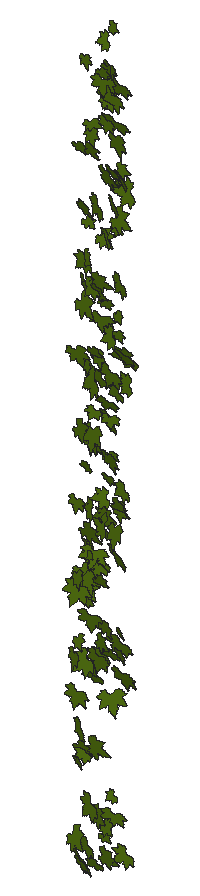
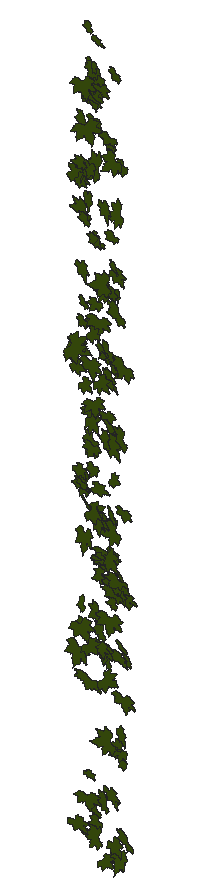
# SketchUp Ruby script. Lengths in inches.
U = 1.inch
M = Sketchup.active_model
def pt(a) = Geom::Point3d.new(a.map { |v| v * U })
def face(e, loops, mat)
  f = e.add_face(loops[0].map { |a| pt(a) })
  loops[1..].each { |l| e.add_face(l.map { |a| pt(a) }).erase! }
  f.material = f.back_material = mat if mat
  f
end
# faces: each face lists its corners as indices into pts; further lists are holes
def faces(e, pts, list, mat = nil) = list.each { |f| face(e, (f[0].is_a?(Array) ? f : [f]).map { |l| l.map { |i| pts[i] } }, mat) }
# xy, xz, yz: faces in a plane at the given z, y or x. An outline is a flat list of corners, or four numbers for a rectangle; further outlines are holes
def ring(l) = l.size == 4 ? [[l[0], l[1]], [l[2], l[1]], [l[2], l[3]], [l[0], l[3]]] : l.each_slice(2).to_a
def flat(e, list, mat, &to3) = list.each { |f| face(e, (f[0].is_a?(Array) ? f : [f]).map { |l| ring(l).map { |u, v| to3.(u, v) } }, mat) }
def xy(e, z, list, mat = nil) = flat(e, list, mat) { |x, y| [x, y, z] }
def xz(e, y, list, mat = nil) = flat(e, list, mat) { |x, z| [x, y, z] }
def yz(e, x, list, mat = nil) = flat(e, list, mat) { |y, z| [x, y, z] }
def lines(e, pts, list) = list.each { |a, b| e.add_line(pt(pts[a]), pt(pts[b])) }
# prism: a flat outline (further loops are holes) pulled along v
def prism(e, loops, v, mat = nil)
  f = face(e, loops, mat); d = Geom::Vector3d.new(v.map { |x| x * U })
  f.pushpull(f.normal.samedirection?(d) ? d.length : -d.length)
end
def box(e, o, s, mat = nil) = prism(e, [[o, [o[0] + s[0], o[1], o[2]], [o[0] + s[0], o[1] + s[1], o[2]], [o[0], o[1] + s[1], o[2]]]], [0, 0, s[2]], mat)
def at(x, y, z, deg = 0) = Geom::Transformation.translation(pt([x, y, z])) * Geom::Transformation.rotation(ORIGIN, Z_AXIS, deg.degrees)
def axes(o, x, y, z) = Geom::Transformation.new([*x, 0, *y, 0, *z, 0, *pt(o).to_a, 1])
def part(name) = M.definitions.add(name)
# library, detail: a bought-in or finely detailed component or shape, given as its bounding box
def library(name, o, s) = part(name).tap { |d| box(d.entities, o, s) }
def detail(e, o, s) = box(e.add_group.entities, o, s)
def put(e, d, t, mat = nil) = e.add_instance(d, t).tap { |i| i.material = mat if mat }
def group(e, t, mat = nil) = e.add_group.tap { |g| g.transformation = t; g.material = mat if mat }.entities
root = M.entities
M.materials.add("[Vegetation Blur 03]").color = [83, 114, 18]
c1 = part("ivy")
xy(c1.entities,0,[[0.782,0,0.786,0,0.787,0.005,0.789,0.009,0.821,0.072,0.875,0.147,1.001,0.272,1.073,0.331,1.137,0.363,1.178,0.379,1.223,0.384,1.272,0.383,1.311,0.374,1.36,0.355,1.399,0.334,1.491,0.285,1.541,0.244,1.583,0.199,1.617,0.15,1.64,0.128,1.662,0.115,1.717,0.105,1.745,0.093,1.784,0.054,1.819,0.057,1.854,0.064,1.882,0.075,1.896,0.074,1.91,0.071,1.937,0.063,1.964,0.053,1.99,0.038,2.016,0.015,2.034,0.002,2.04,0,2.038,0.003,2.036,0.007,2.033,0.038,2.036,0.068,2.045,0.1,2.055,0.116,2.064,0.123,2.077,0.129,2.088,0.129,2.106,0.132,2.118,0.13,2.179,0.132,2.207,0.133,2.225,0.133,2.242,0.138,2.22,0.162,2.207,0.186,2.206,0.213,2.212,0.236,2.228,0.262,2.247,0.274,2.298,0.283,2.355,0.294,2.37,0.296,2.376,0.295,2.377,0.3,2.377,0.303,2.385,0.329,2.411,0.37,2.426,0.392,2.449,0.407,2.511,0.426,2.561,0.444,2.619,0.466,2.589,0.469,2.561,0.476,2.501,0.5,2.449,0.516,2.424,0.523,2.401,0.535,2.377,0.556,2.372,0.568,2.36,0.575,2.268,0.586,2.225,0.592,2.207,0.599,2.194,0.61,2.143,0.65,2.13,0.664,2.122,0.682,2.123,0.7,2.13,0.719,2.148,0.75,2.17,0.781,2.195,0.807,2.221,0.828,2.284,0.874,2.291,0.88,2.288,0.887,2.276,0.9,2.267,0.916,2.265,0.933,2.273,0.967,2.292,1.002,2.313,1.03,2.334,1.054,2.348,1.067,2.358,1.074,2.363,1.076,2.362,1.081,2.35,1.094,2.347,1.11,2.35,1.143,2.359,1.18,2.385,1.254,2.415,1.324,2.448,1.393,2.45,1.4,2.446,1.398,2.44,1.394,2.427,1.383,2.402,1.36,2.376,1.339,2.345,1.324,2.305,1.309,2.282,1.303,2.273,1.306,2.245,1.294,2.212,1.287,2.187,1.291,2.163,1.301,2.142,1.316,2.134,1.327,2.124,1.325,2.09,1.292,2.053,1.259,2.014,1.234,1.973,1.215,1.954,1.21,1.931,1.208,1.909,1.212,1.893,1.22,1.879,1.233,1.872,1.248,1.867,1.281,1.864,1.319,1.821,1.258,1.773,1.197,1.726,1.141,1.698,1.121,1.679,1.116,1.666,1.117,1.647,1.122,1.632,1.129,1.62,1.141,1.617,1.154,1.617,1.219,1.621,1.254,1.623,1.268,1.623,1.281,1.618,1.314,1.606,1.346,1.603,1.375,1.607,1.403,1.603,1.467,1.599,1.499,1.605,1.525,1.614,1.552,1.629,1.577,1.635,1.589,1.629,1.587,1.618,1.582,1.596,1.566,1.581,1.556,1.568,1.552,1.557,1.55,1.545,1.553,1.531,1.562,1.522,1.572,1.504,1.591,1.486,1.611,1.474,1.631,1.457,1.666,1.455,1.684,1.457,1.698,1.452,1.715,1.444,1.728,1.424,1.754,1.419,1.772,1.423,1.786,1.434,1.819,1.444,1.848,1.446,1.855,1.44,1.861,1.43,1.867,1.386,1.904,1.349,1.948,1.326,1.973,1.31,1.995,1.288,2.048,1.284,2.153,1.287,2.254,1.284,2.255,1.282,2.253,1.278,2.247,1.274,2.237,1.266,2.216,1.226,2.125,1.208,2.076,1.184,2.033,1.155,1.984,1.135,1.942,1.111,1.899,1.083,1.861,1.053,1.85,1.059,1.83,1.061,1.809,1.056,1.79,1.049,1.767,1.04,1.749,1.018,1.733,0.994,1.726,0.942,1.734,0.95,1.6875,0.944,1.645,0.932,1.608,0.911,1.585,0.881,1.58,0.854,1.582,0.828,1.588,0.785,1.618,0.773,1.625,0.775,1.614,0.779,1.598,0.796,1.502,0.818,1.402,0.861,1.283,0.882,1.224,0.894,1.174,0.892,1.148,0.886,1.123,0.881,1.107,0.872,1.099,0.849,1.094,0.818,1.092,0.789,1.098,0.762,1.107,0.753,1.113,0.721,1.139,0.698,1.163,0.678,1.194,0.665,1.224,0.628,1.28,0.612,1.312,0.606,1.327,0.606,1.314,0.599,1.282,0.594,1.267,0.581,1.256,0.544,1.245,0.512,1.244,0.473,1.249,0.444,1.256,0.382,1.288,0.339,1.306,0.324,1.316,0.317,1.324,0.309,1.326,0.27,1.314,0.227,1.313,0.185,1.3125,0.152,1.317,0.122,1.328,0.092,1.345,0.073,1.353,0.079,1.338,0.092,1.308,0.117,1.249,0.13,1.215,0.139,1.164,0.147,1.148,0.157,1.136,0.163,1.122,0.174,1.086,0.177,1.067,0.182,1.054,0.186,1.043,0.191,1.038,0.211,1.028,0.237,1.005,0.25,0.974,0.253,0.96,0.25,0.944,0.242,0.914,0.243,0.906,0.249,0.902,0.26,0.894,0.289,0.88,0.307,0.873,0.322,0.862,0.364,0.799,0.403,0.738,0.431,0.709,0.439,0.691,0.441,0.678,0.4375,0.66,0.428,0.645,0.394,0.623,0.303,0.594,0.255,0.581,0.214,0.577,0.179,0.573,0.173,0.568,0.175,0.561,0.167,0.55,0.141,0.523,0.113,0.503,0.077,0.49,0.045,0.486,0.026,0.485,0.019,0.486,0.011,0.483,0,0.471,0.014,0.467,0.044,0.455,0.058,0.447,0.07,0.438,0.097,0.411,0.125,0.394,0.158,0.377,0.174,0.366,0.182,0.359,0.185,0.361,0.242,0.331,0.253,0.316,0.258,0.303,0.262,0.283,0.274,0.278,0.308,0.274,0.341,0.252,0.366,0.226,0.366,0.222,0.37,0.22,0.38,0.221,0.395,0.221,0.425,0.216,0.45,0.207,0.465,0.192,0.473,0.178,0.484,0.15,0.489,0.116,0.483,0.089,0.468,0.058,0.45,0.035,0.435,0.018,0.429,0.011,0.434,0.012,0.438,0.014,0.469,0.019,0.542,0.016,0.581,0.015,0.612,0.027,0.68,0.055,0.696,0.057,0.712,0.052,0.73,0.045,0.741,0.036,0.766,0.014]])
put(root,c1,axes([72.84,173.7,61.72],[0.32192,-0.21102,-0.29136],[-0.33943,0.22769,-0.27574],[-0.15085,-0.96265,-0.00135]),"[Vegetation Blur 03]")
put(root,c1,axes([72.2,173.7,63.29],[0.58789,-0.11281,-0.04556],[-0.05859,-0.05769,-0.48112],[-0.05185,-1.21383,0.0271]),"[Vegetation Blur 03]")
put(root,c1,axes([72.33,173.7,72.92],[0.43658,-0.10423,0.00392],[0.00224,-0.04583,-0.35826],[-0.05083,-0.89729,0.01784]),"[Vegetation Blur 03]")
put(root,c1,axes([72.26,173.7,68.72],[0.62885,-0.10059,-0.07918],[-0.103,-0.17922,-0.50906],[-0.03454,-1.29703,0.07648]),"[Vegetation Blur 03]")
put(root,c1,axes([72.38,173.7,65.2],[0.43914,-0.29657,0.03896],[0.03337,-0.10478,-0.37595],[-0.14811,-0.90294,0.03083]),"[Vegetation Blur 03]")
put(root,c1,axes([72.09,173.7,55.21],[0.24806,0.03915,0.43187],[0.51673,-0.28046,-0.19369],[-0.11561,-1.16947,0.06091]),"[Vegetation Blur 03]")
put(root,c1,axes([72.89,173.7,68.78],[0.30881,-0.07275,-0.21101],[-0.25864,0.02403,-0.25343],[-0.03462,-0.82843,0.01118]),"[Vegetation Blur 03]")
put(root,c1,axes([72.42,173.7,90.69],[0.29342,-0.08692,0.17033],[0.21238,0.06683,-0.23833],[-0.01533,-0.73794,-0.04165]),"[Vegetation Blur 03]")
put(root,c1,axes([72.03,173.7,80.21],[0.52256,-0.08904,0.24501],[0.30058,-0.01277,-0.42774],[-0.04062,-1.24009,-0.01319]),"[Vegetation Blur 03]")
put(root,c1,axes([72.53,173.7,59.625],[0.27556,-0.19726,0.13683],[0.17351,-0.01114,-0.23526],[-0.08482,-0.66366,-0.03672]),"[Vegetation Blur 03]")
put(root,c1,axes([72.5,173.7,65.52],[0.23663,-0.00308,0.21961],[0.25991,-0.18831,-0.18695],[-0.06967,-0.71292,0.04843]),"[Vegetation Blur 03]")
put(root,c1,axes([73.38,173.7,74.76],[0.04516,0.08728,-0.24004],[-0.29622,0.06188,-0.03358],[-0.02362,-0.6092,-0.0378]),"[Vegetation Blur 03]")
put(root,c1,axes([72.97,173.7,85.52],[0.38178,-0.11889,-0.25625],[-0.31299,0.05919,-0.31491],[-0.06294,-1.01546,0.01165]),"[Vegetation Blur 03]")
put(root,c1,axes([73.13,173.7,55.86],[0.3336,-0.07994,-0.30777],[-0.37102,0.14358,-0.27372],[-0.07791,-1.02608,-0.01433]),"[Vegetation Blur 03]")
put(root,c1,axes([73.05,173.7,84.32],[0.23472,-0.16453,-0.13977],[-0.15775,0.13898,-0.20218],[-0.10411,-0.58153,-0.00877]),"[Vegetation Blur 03]")
put(root,c1,axes([72.51,173.7,68.86],[0.29156,-0.09126,0.22735],[0.25627,-0.25873,-0.23525],[-0.11785,-0.78843,0.05088]),"[Vegetation Blur 03]")
put(root,c1,axes([73.09,173.7,60.46],[0.296,-0.08214,-0.20649],[-0.25613,-0.08908,-0.23898],[-0.00188,-0.79632,0.04803]),"[Vegetation Blur 03]")
put(root,c1,axes([72.64,173.7,54.66],[0.4103,-0.202,-0.00421],[0.00893,0.12198,-0.34084],[-0.09789,-0.83552,-0.04874]),"[Vegetation Blur 03]")
put(root,c1,axes([72.49,173.7,55.04],[0.61856,-0.3329,-0.06965],[-0.05285,0.26763,-0.51381],[-0.1751,-1.25675,-0.09097]),"[Vegetation Blur 03]")
put(root,c1,axes([72.36,173.7,69.02],[0.386,0.08915,0.27036],[0.33331,-0.03157,-0.31533],[0.02283,-1.04625,0.03255]),"[Vegetation Blur 03]")
put(root,c1,axes([72.46,173.7,60.09],[0.30498,-0.11066,0.28031],[0.34736,0.05892,-0.24807],[-0.01408,-0.94337,-0.04838]),"[Vegetation Blur 03]")
put(root,c1,axes([73.375,173.7,76.82],[0.38094,-0.16652,-0.42659],[-0.51102,0.22607,-0.31784],[-0.13644,-1.3116,-0.00062]),"[Vegetation Blur 03]")
put(root,c1,axes([73.51,173.7,70.9375],[0.2944,-0.05147,-0.44172],[-0.52796,0.2576,-0.2391],[-0.12176,-1.24142,-0.0313]),"[Vegetation Blur 03]")
put(root,c1,axes([73.69,173.7,72.95],[0.09708,-0.16375,-0.35064],[-0.41312,0.26056,-0.09533],[-0.14231,-0.86813,0.03753]),"[Vegetation Blur 03]")
put(root,c1,axes([72.49,173.7,75.99],[0.19561,-0.07372,0.44835],[0.54629,-0.12238,-0.16192],[-0.06809,-1.19373,-0.01109]),"[Vegetation Blur 03]")
put(root,c1,axes([73.72,173.7,64.41],[0.11047,0.20453,-0.35161],[-0.44126,-0.0065,-0.09294],[0.02783,-0.9152,-0.07792]),"[Vegetation Blur 03]")
put(root,c1,axes([73.12,173.7,65.54],[0.50163,-0.24569,-0.26541],[-0.34021,-0.12729,-0.40976],[-0.06534,-1.2236,0.09592]),"[Vegetation Blur 03]")
put(root,c1,axes([72.3,173.7,68.8125],[0.58138,0.04851,0.24502],[0.30111,-0.07156,-0.47365],[0.00495,-1.34457,0.03405]),"[Vegetation Blur 03]")
put(root,c1,axes([72.89,173.7,95.36],[0.32177,-0.10077,0.13804],[0.16444,-0.08743,-0.26534],[-0.06299,-0.74292,0.0125]),"[Vegetation Blur 03]")
put(root,c1,axes([72.95,173.7,86.86],[0.2013,0.04338,0.20783],[0.25534,-0.0094,-0.16443],[0.00948,-0.6679,0.01581]),"[Vegetation Blur 03]")
put(root,c1,axes([73.01,173.7,70.22],[0.28684,-0.06236,0.1063],[0.12625,-0.08285,-0.23456],[-0.04409,-0.64295,0.01992]),"[Vegetation Blur 03]")
put(root,c1,axes([72.66,173.7,68.17],[0.3314,0.11464,0.31783],[0.39311,-0.13672,-0.26526],[-0.0151,-1.04335,0.06968]),"[Vegetation Blur 03]")
put(root,c1,axes([73.1,173.7,67.56],[0.07858,-0.01385,0.24493],[0.29907,-0.05144,-0.06436],[-0.02588,-0.6363,-0.00013]),"[Vegetation Blur 03]")
put(root,c1,axes([73.67,173.7,54.8125],[0.1696,0.1381,-0.24942],[-0.31204,0.02191,-0.13942],[0.02307,-0.7189,-0.05216]),"[Vegetation Blur 03]")
put(root,c1,axes([73.0625,173.7,84.93],[0.07908,0.01608,0.29029],[0.3424,-0.20709,-0.06032],[-0.09663,-0.72064,0.02381]),"[Vegetation Blur 03]")
put(root,c1,axes([72.54,173.7,82.52],[0.31957,-0.02324,0.46113],[0.55443,-0.24575,-0.25788],[-0.10943,-1.31297,0.04011]),"[Vegetation Blur 03]")
put(root,c1,axes([72.82,173.7,67.3],[0.62015,-0.02976,-0.03519],[-0.04222,0.07375,-0.50547],[-0.01689,-1.27709,-0.02837]),"[Vegetation Blur 03]")
put(root,c1,axes([73.05,173.7,79.85],[0.25768,-0.12141,0.16925],[0.19637,-0.14245,-0.21521],[-0.08903,-0.66558,0.01519]),"[Vegetation Blur 03]")
put(root,c1,axes([72.72,173.7,90.72],[0.41952,-0.13561,0.24997],[0.31292,0.12999,-0.33871],[-0.01528,-1.06095,-0.07345]),"[Vegetation Blur 03]")
put(root,c1,axes([72.75,173.7,87.72],[0.30187,-0.29092,0.34167],[0.43037,-0.04293,-0.25902],[-0.10016,-1.06123,-0.08319]),"[Vegetation Blur 03]")
put(root,c1,axes([73.3,173.7,58.22],[0.52518,-0.29878,-0.23016],[-0.2856,0.04291,-0.44284],[-0.13799,-1.22592,0.0406]),"[Vegetation Blur 03]")
put(root,c1,axes([73.53,173.7,79.49],[0.2496,-0.10992,-0.13236],[-0.16418,0.00788,-0.20725],[-0.04691,-0.61248,0.02109]),"[Vegetation Blur 03]")
put(root,c1,axes([73.4,173.7,84.38],[0.42696,-0.16855,-0.18226],[-0.22665,-0.00186,-0.3534],[-0.07216,-0.99152,0.03164]),"[Vegetation Blur 03]")
put(root,c1,axes([73.42,173.7,77.82],[0.33208,0.00162,-0.09351],[-0.114,-0.06757,-0.26985],[0.01145,-0.71971,0.02513]),"[Vegetation Blur 03]")
put(root,c1,axes([73.05,173.7,92.02],[0.3458,0.03513,0.16386],[0.2014,-0.03386,-0.28195],[0.00648,-0.82214,0.01861]),"[Vegetation Blur 03]")
put(root,c1,axes([73.66,173.7,80.05],[0.48032,-0.40321,-0.3461],[-0.42858,0.11763,-0.41773],[-0.18586,-1.31325,0.06885]),"[Vegetation Blur 03]")
put(root,c1,axes([73.09,173.7,70.63],[0.56687,0.06013,-0.01984],[-0.01943,-0.18427,-0.45761],[0.03267,-1.15295,0.0721]),"[Vegetation Blur 03]")
put(root,c1,axes([73.99,173.7,79.74],[0.21346,0.05085,-0.33078],[-0.40485,0.09932,-0.17162],[-0.03132,-0.93739,-0.03613]),"[Vegetation Blur 03]")
put(root,c1,axes([72.84,173.7,71.1],[0.31154,-0.18802,0.42817],[0.53015,-0.00865,-0.25753],[-0.0503,-1.25557,-0.06234]),"[Vegetation Blur 03]")
put(root,c1,axes([73.16,173.7,91.62],[0.34903,-0.06561,0.18456],[0.21828,-0.15404,-0.28357],[-0.06714,-0.84183,0.0375]),"[Vegetation Blur 03]")
put(root,c1,axes([73.5,173.7,64.33],[0.10915,-0.09215,0.23401],[0.27778,-0.14927,-0.09555],[-0.08399,-0.61343,-0.0119]),"[Vegetation Blur 03]")
put(root,c1,axes([74.52,173.7,72.7],[0.10352,-0.20906,-0.49577],[-0.59692,0.27823,-0.10147],[-0.15173,-1.23717,0.06096]),"[Vegetation Blur 03]")
put(root,c1,axes([73.71,173.7,88.71],[0.46455,-0.28541,-0.24702],[-0.29064,0.17394,-0.39567],[-0.16241,-1.12761,0.00149]),"[Vegetation Blur 03]")
put(root,c1,axes([73.13,173.7,60.02],[0.20638,-0.06433,0.46905],[0.57546,0.04752,-0.16762],[0.01121,-1.25569,-0.03037]),"[Vegetation Blur 03]")
put(root,c1,axes([73.28,173.7,80.62],[0.36896,-0.184,0.21842],[0.27276,0.00042,-0.30684],[-0.07226,-0.93795,-0.04299]),"[Vegetation Blur 03]")
put(root,c1,axes([73.51,173.7,70.04],[0.4452,0.01529,-0.01974],[-0.02317,-0.10578,-0.36101],[0.01016,-0.91136,0.04157]),"[Vegetation Blur 03]")
put(root,c1,axes([73.41,173.7,65.57],[0.60359,-0.16861,-0.0634],[-0.07511,0.04962,-0.497],[-0.08431,-1.25133,-0.01117]),"[Vegetation Blur 03]")
put(root,c1,axes([73.75,173.7,65.6875],[0.43906,-0.08807,-0.12908],[-0.15747,0.03053,-0.36003],[-0.0453,-0.95985,0.00039]),"[Vegetation Blur 03]")
put(root,c1,axes([73.56,173.7,75.65],[0.09017,-0.06413,0.35822],[0.42718,-0.20848,-0.07749],[-0.10559,-0.89821,-0.00759]),"[Vegetation Blur 03]")
put(root,c1,axes([73.48,173.7,82.61],[0.54749,0.01991,-0.01395],[-0.01748,0.04635,-0.4465],[0.00896,-1.12621,-0.01862]),"[Vegetation Blur 03]")
put(root,c1,axes([74.51,173.7,72.92],[0.16632,0.09986,-0.39596],[-0.48659,-0.03313,-0.13745],[0.03103,-1.05488,-0.03317]),"[Vegetation Blur 03]")
put(root,c1,axes([74.19,173.7,70.375],[0.23314,-0.02071,-0.23083],[-0.28282,0.0106,-0.19042],[-0.01038,-0.7542,0.00366]),"[Vegetation Blur 03]")
put(root,c1,axes([74.01,173.7,72.26],[0.37136,-0.15214,-0.22354],[-0.25515,0.22677,-0.30661],[-0.12403,-0.92207,-0.03852]),"[Vegetation Blur 03]")
put(root,c1,axes([73.21,173.7,76.85],[0.61028,-0.27277,0.17175],[0.18054,-0.30337,-0.50308],[-0.17106,-1.2933,0.08178]),"[Vegetation Blur 03]")
put(root,c1,axes([74.41,173.7,77.78],[0.25339,0.01902,-0.3994],[-0.47391,0.29322,-0.19806],[-0.12245,-1.09547,-0.05995]),"[Vegetation Blur 03]")
put(root,c1,axes([73.61,173.7,68.9],[0.22705,-0.08947,0.23456],[0.29067,0.06726,-0.18337],[-0.00101,-0.75069,-0.04439]),"[Vegetation Blur 03]")
put(root,c1,axes([73.92,173.7,78.45],[0.41502,0.09791,-0.15811],[-0.19925,0.15826,-0.33295],[0.0098,-0.92912,-0.07337]),"[Vegetation Blur 03]")
put(root,c1,axes([74.49,173.7,73.94],[0.1638,-0.10041,-0.33523],[-0.41333,-0.07495,-0.13099],[0.01603,-0.90688,0.04794]),"[Vegetation Blur 03]")
put(root,c1,axes([73.47,173.7,83.78],[0.15315,-0.11376,0.42127],[0.51825,0.09795,-0.12133],[0.03021,-1.10363,-0.05419]),"[Vegetation Blur 03]")
put(root,c1,axes([74.45,173.7,87.02],[0.17953,-0.09504,-0.30608],[-0.36446,0.18198,-0.15128],[-0.09974,-0.83603,0.00186]),"[Vegetation Blur 03]")
put(root,c1,axes([74.57,173.7,82.08],[0.09179,0.09251,-0.29251],[-0.35994,0.08732,-0.07089],[-0.03033,-0.7563,-0.04396]),"[Vegetation Blur 03]")
put(root,c1,axes([73.61,173.7,56.72],[0.09186,-0.01547,0.40746],[0.48625,-0.23456,-0.07442],[-0.11344,-1.01793,0.01096]),"[Vegetation Blur 03]")
put(root,c1,axes([73.66,173.7,83.4],[0.10455,-0.16948,0.36645],[0.45413,-0.0579,-0.09052],[-0.04648,-0.94693,-0.06005]),"[Vegetation Blur 03]")
put(root,c1,axes([73.55,173.7,80.5],[0.35673,-0.12377,0.22075],[0.25958,-0.16822,-0.29423],[-0.09696,-0.90576,0.02448]),"[Vegetation Blur 03]")
put(root,c1,axes([73.58,173.7,94.68],[0.55862,-0.01173,0.01902],[0.02312,-0.03492,-0.45573],[-0.0064,-1.15001,0.01364]),"[Vegetation Blur 03]")
put(root,c1,axes([73.77,173.7,94.86],[0.27413,-0.06194,0.16545],[0.20434,0.02916,-0.2238],[-0.01572,-0.70099,-0.02393]),"[Vegetation Blur 03]")
put(root,c1,axes([74.52,173.7,65.8],[0.1902,0.17643,-0.26649],[-0.33646,0.03567,-0.15623],[0.02775,-0.7768,-0.0677]),"[Vegetation Blur 03]")
put(root,c1,axes([73.88,173.7,83.2],[0.28384,0.00263,0.11756],[0.14245,0.09199,-0.22943],[0.02136,-0.64851,-0.03207]),"[Vegetation Blur 03]")
put(root,c1,axes([73.78,173.7,65.66],[0.12722,-0.05638,0.35512],[0.42991,-0.13892,-0.10606],[-0.07252,-0.92248,-0.00573]),"[Vegetation Blur 03]")
put(root,c1,axes([74.54,173.7,97.1875],[0.2034,-0.19719,-0.25526],[-0.32297,-0.00076,-0.17132],[-0.05192,-0.76775,0.06573]),"[Vegetation Blur 03]")
put(root,c1,axes([73.72,173.7,86.24],[0.23996,0.10055,0.29847],[0.36879,-0.09254,-0.19259],[-0.01117,-0.89532,0.05342]),"[Vegetation Blur 03]")
put(root,c1,axes([73.92,173.7,56.02],[0.1988,-0.0106,0.20658],[0.25313,-0.00387,-0.16228],[-0.00466,-0.6623,-0.00236]),"[Vegetation Blur 03]")
put(root,c1,axes([74.29,173.7,92.93],[0.48948,0.16058,-0.27855],[-0.34964,0.16113,-0.39462],[0.01829,-1.21733,-0.08898]),"[Vegetation Blur 03]")
put(root,c1,axes([74.07,173.7,92.77],[0.4277,-0.13208,-0.01923],[-0.02433,-0.00684,-0.35292],[-0.0639,-0.88143,0.00562]),"[Vegetation Blur 03]")
put(root,c1,axes([74.15,173.7,74.61],[0.33381,-0.09287,0.01816],[0.028,0.08748,-0.27236],[-0.04181,-0.68286,-0.03736]),"[Vegetation Blur 03]")
put(root,c1,axes([74,173.7,56.45],[0.18478,0.02807,0.2907],[0.35178,-0.14758,-0.1467],[-0.05752,-0.81244,0.03669]),"[Vegetation Blur 03]")
put(root,c1,axes([74.02,173.7,75.66],[0.39754,-0.01789,0.09307],[0.11433,0.03939,-0.32408],[-0.00307,-0.85015,-0.01697]),"[Vegetation Blur 03]")
put(root,c1,axes([73.92,173.7,66.79],[0.32691,-0.16543,0.24576],[0.30294,-0.04245,-0.2729],[-0.07327,-0.91364,-0.03182]),"[Vegetation Blur 03]")
put(root,c1,axes([74.15,173.7,77.57],[0.37993,0.04432,0.03279],[0.04106,-0.03097,-0.31026],[0.01982,-0.78558,0.01408]),"[Vegetation Blur 03]")
put(root,c1,axes([74.0625,173.7,95.3125],[0.38821,-0.11193,0.10755],[0.13579,0.05066,-0.31818],[-0.04343,-0.84212,-0.03344]),"[Vegetation Blur 03]")
put(root,c1,axes([74.22,173.7,94.46],[0.60025,-0.11632,-0.20653],[-0.25299,0.02521,-0.49198],[-0.05685,-1.34025,0.00867]),"[Vegetation Blur 03]")
put(root,c1,axes([74.16,173.7,80.3],[0.58763,-0.14391,-0.14762],[-0.17735,0.08172,-0.48275],[-0.07846,-1.26257,-0.01442]),"[Vegetation Blur 03]")
put(root,c1,axes([74.74,173.7,82.34],[0.30417,-0.25351,-0.27604],[-0.3464,0.04167,-0.26026],[-0.0979,-0.93513,0.06323]),"[Vegetation Blur 03]")
put(root,c1,axes([73.97,173.7,93.55],[0.34233,0.0367,0.25351],[0.30852,-0.16299,-0.27378],[-0.04025,-0.93715,0.05755]),"[Vegetation Blur 03]")
put(root,c1,axes([74.19,173.7,57.64],[0.52025,0.05923,-0.06815],[-0.08303,-0.02209,-0.42521],[0.03012,-1.08405,0.00494]),"[Vegetation Blur 03]")
put(root,c1,axes([74.03,173.7,54.73],[0.10484,-0.11239,0.45286],[0.55605,-0.06423,-0.08825],[-0.04094,-1.16025,-0.03898]),"[Vegetation Blur 03]")
put(root,c1,axes([74.28,173.7,95.62],[0.38177,-0.16884,0.00908],[0.01686,0.05275,-0.31784],[-0.08106,-0.78418,-0.02334]),"[Vegetation Blur 03]")
put(root,c1,axes([74.36,173.7,90.35],[0.38893,-0.1332,-0.05202],[-0.05011,0.16639,-0.31658],[-0.07577,-0.79377,-0.05763]),"[Vegetation Blur 03]")
put(root,c1,axes([74.95,173.7,79.25],[0.18993,0.03098,-0.27697],[-0.33885,0.07408,-0.15347],[-0.02412,-0.79685,-0.02503]),"[Vegetation Blur 03]")
put(root,c1,axes([74.75,173.7,58.74],[0.21979,-0.07452,-0.15702],[-0.1954,-0.04663,-0.1787],[-0.01213,-0.59927,0.03343]),"[Vegetation Blur 03]")
put(root,c1,axes([74.62,173.7,88.88],[0.36908,-0.2283,-0.18774],[-0.2052,0.23015,-0.31272],[-0.15204,-0.86483,-0.03366]),"[Vegetation Blur 03]")
put(root,c1,axes([74.53,173.7,94.97],[0.53586,0.00327,-0.21137],[-0.25728,0.14717,-0.4341],[-0.0297,-1.21585,-0.05311]),"[Vegetation Blur 03]")
put(root,c1,axes([74.54,173.7,97.14],[0.05613,0.01305,0.23736],[0.28926,-0.0672,-0.04498],[-0.03088,-0.6058,0.0101]),"[Vegetation Blur 03]")
put(root,c1,axes([73.87,173.7,63.34],[0.58242,0.07305,0.2372],[0.29248,-0.20649,-0.46835],[-0.01349,-1.32342,0.08617]),"[Vegetation Blur 03]")
put(root,c1,axes([74.73,173.7,66.7],[0.47827,0.03325,-0.27343],[-0.33498,0.10885,-0.38819],[-0.01718,-1.19669,-0.04291]),"[Vegetation Blur 03]")
put(root,c1,axes([74.07,173.7,75.72],[0.52923,-0.27231,0.14829],[0.19148,0.04522,-0.44212],[-0.11773,-1.15056,-0.05247]),"[Vegetation Blur 03]")
put(root,c1,axes([74.23,173.7,89.39],[0.07798,-0.22712,0.49701],[0.61066,-0.17712,-0.07655],[-0.10063,-1.25091,-0.0794]),"[Vegetation Blur 03]")
put(root,c1,axes([75.27,173.7,89.81],[0.1507,0.00007,-0.27274],[-0.3307,0.10871,-0.1217],[-0.04814,-0.74651,-0.01775]),"[Vegetation Blur 03]")
put(root,c1,axes([74.54,173.7,71.22],[0.58057,-0.26082,-0.16045],[-0.16911,0.27993,-0.47915],[-0.16161,-1.22989,-0.07503]),"[Vegetation Blur 03]")
put(root,c1,axes([75.72,173.7,81.36],[0.08849,0.22325,-0.50781],[-0.6312,-0.01504,-0.0743],[0.02262,-1.29319,-0.0868]),"[Vegetation Blur 03]")
put(root,c1,axes([74.65,173.7,87.03],[0.11812,0.02268,0.27727],[0.33763,-0.09352,-0.0946],[-0.03936,-0.73423,0.02061]),"[Vegetation Blur 03]")
put(root,c1,axes([74.99,173.7,85.14],[0.45147,-0.25025,-0.22719],[-0.26949,0.14362,-0.38159],[-0.1402,-1.08195,0.00189]),"[Vegetation Blur 03]")
put(root,c1,axes([74.75,173.7,81.9],[0.26219,-0.05379,0.13773],[0.16863,-0.0189,-0.21498],[-0.02696,-0.64136,-0.00522]),"[Vegetation Blur 03]")
put(root,c1,axes([74.92,173.7,90.26],[0.41315,-0.18544,-0.14251],[-0.1576,0.18691,-0.3426],[-0.11735,-0.90388,-0.04161]),"[Vegetation Blur 03]")
put(root,c1,axes([74.79,173.7,82.78],[0.19571,-0.04059,0.18321],[0.21938,-0.10557,-0.15978],[-0.05153,-0.6037,0.01562]),"[Vegetation Blur 03]")
put(root,c1,axes([75.29,173.7,74.61],[0.30292,-0.11557,-0.26319],[-0.32214,0.05514,-0.25077],[-0.05807,-0.90879,0.01825]),"[Vegetation Blur 03]")
put(root,c1,axes([74.88,173.7,73.49],[0.2893,-0.06946,0.05279],[0.06075,-0.07196,-0.23668],[-0.04039,-0.60575,0.02206]),"[Vegetation Blur 03]")
put(root,c1,axes([74.92,173.7,89.93],[0.04916,0.02287,0.27993],[0.3427,0.03405,-0.04052],[0.01796,-0.71221,0.00705]),"[Vegetation Blur 03]")
put(root,c1,axes([74.87,173.7,81.14],[0.46406,-0.05319,-0.06714],[-0.07481,0.21257,-0.37089],[-0.04289,-0.94624,-0.07954]),"[Vegetation Blur 03]")
put(root,c1,axes([75.86,173.7,80.08],[0.07216,-0.07343,-0.39325],[-0.48158,0.07012,-0.06092],[-0.03906,-1.00014,0.0246]),"[Vegetation Blur 03]")
put(root,c1,axes([75.3,173.7,56.21],[0.3982,-0.07833,-0.27853],[-0.34327,-0.06231,-0.32413],[-0.0091,-1.07738,0.039]),"[Vegetation Blur 03]")
put(root,c1,axes([74.58,173.7,87.25],[0.15618,0.05581,0.47785],[0.58342,-0.13447,-0.12454],[-0.05625,-1.2397,0.03502]),"[Vegetation Blur 03]")
put(root,c1,axes([75.91,173.7,90.125],[0.18243,-0.13935,-0.48722],[-0.59996,0.02639,-0.15082],[-0.03212,-1.28429,0.04976]),"[Vegetation Blur 03]")
put(root,c1,axes([74.6,173.7,72.21],[0.50493,-0.24622,0.19162],[0.19585,-0.34808,-0.41408],[-0.17632,-1.09173,0.08881]),"[Vegetation Blur 03]")
put(root,c1,axes([74.79,173.7,73.33],[0.43109,-0.16307,0.09857],[0.11374,-0.09903,-0.3571],[-0.08905,-0.91592,0.02106]),"[Vegetation Blur 03]")
put(root,c1,axes([74.875,173.7,65.92],[0.34195,-0.22556,0.12659],[0.16367,0.01646,-0.28987],[-0.09636,-0.7725,-0.04314]),"[Vegetation Blur 03]")
put(root,c1,axes([75.03,173.7,66.86],[0.1642,-0.18374,0.20113],[0.24769,-0.08699,-0.14719],[-0.08574,-0.60314,-0.04004]),"[Vegetation Blur 03]")
put(root,c1,axes([74.5,173.7,92.07],[0.58958,-0.29849,0.19052],[0.22934,-0.09222,-0.49546],[-0.15145,-1.30163,-0.00859]),"[Vegetation Blur 03]")
put(root,c1,axes([74.66,173.7,65.01],[0.64437,-0.16461,0.01325],[0.02704,0.17964,-0.52482],[-0.07702,-1.31419,-0.0734]),"[Vegetation Blur 03]")
put(root,c1,axes([74.71,173.7,72.94],[0.20255,-0.18759,0.41357],[0.50926,-0.09194,-0.17269],[-0.07578,-1.11921,-0.05513]),"[Vegetation Blur 03]")
